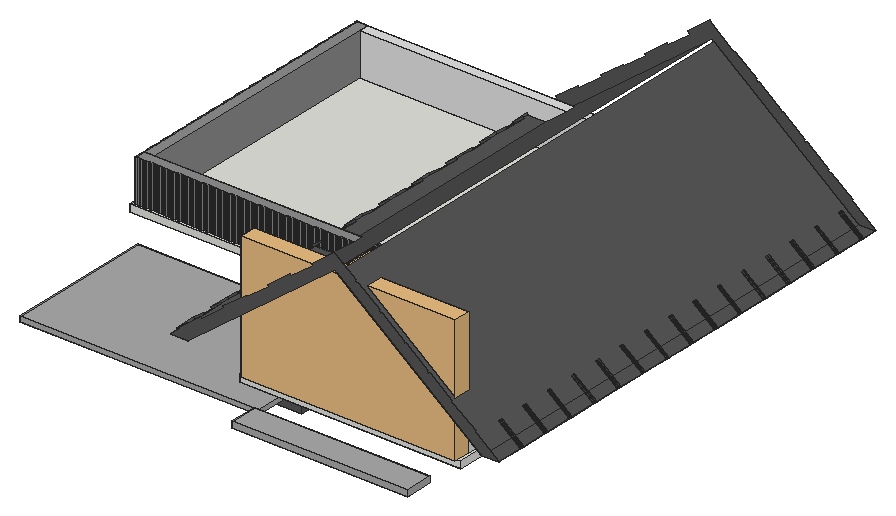
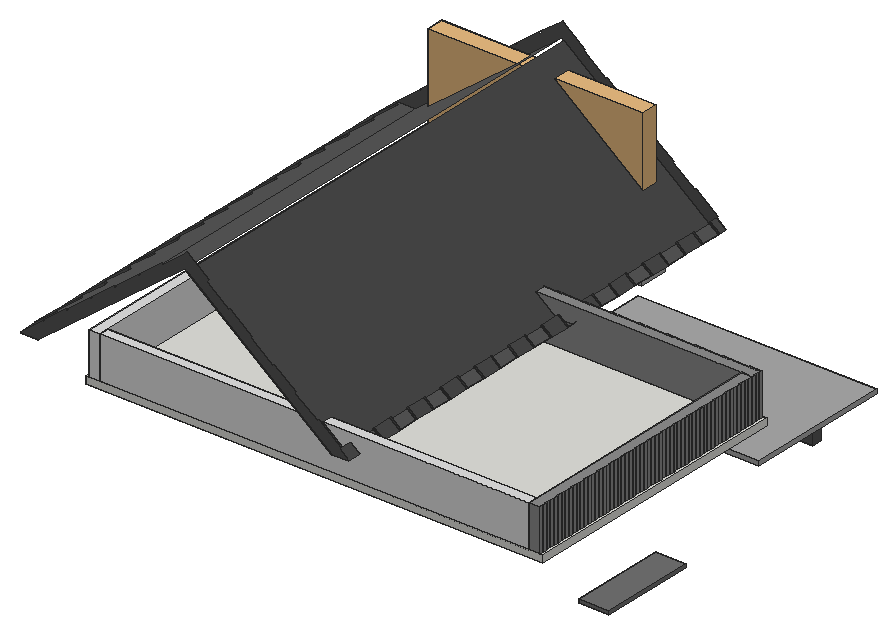
# SketchUp Ruby script. Lengths in inches.
U = 1.inch
M = Sketchup.active_model
def pt(a) = Geom::Point3d.new(a.map { |v| v * U })
def face(e, loops, mat)
  f = e.add_face(loops[0].map { |a| pt(a) })
  loops[1..].each { |l| e.add_face(l.map { |a| pt(a) }).erase! }
  f.material = f.back_material = mat if mat
  f
end
# faces: each face lists its corners as indices into pts; further lists are holes
def faces(e, pts, list, mat = nil) = list.each { |f| face(e, (f[0].is_a?(Array) ? f : [f]).map { |l| l.map { |i| pts[i] } }, mat) }
# xy, xz, yz: faces in a plane at the given z, y or x. An outline is a flat list of corners, or four numbers for a rectangle; further outlines are holes
def ring(l) = l.size == 4 ? [[l[0], l[1]], [l[2], l[1]], [l[2], l[3]], [l[0], l[3]]] : l.each_slice(2).to_a
def flat(e, list, mat, &to3) = list.each { |f| face(e, (f[0].is_a?(Array) ? f : [f]).map { |l| ring(l).map { |u, v| to3.(u, v) } }, mat) }
def xy(e, z, list, mat = nil) = flat(e, list, mat) { |x, y| [x, y, z] }
def xz(e, y, list, mat = nil) = flat(e, list, mat) { |x, z| [x, y, z] }
def yz(e, x, list, mat = nil) = flat(e, list, mat) { |y, z| [x, y, z] }
def lines(e, pts, list) = list.each { |a, b| e.add_line(pt(pts[a]), pt(pts[b])) }
# prism: a flat outline (further loops are holes) pulled along v
def prism(e, loops, v, mat = nil)
  f = face(e, loops, mat); d = Geom::Vector3d.new(v.map { |x| x * U })
  f.pushpull(f.normal.samedirection?(d) ? d.length : -d.length)
end
def box(e, o, s, mat = nil) = prism(e, [[o, [o[0] + s[0], o[1], o[2]], [o[0] + s[0], o[1] + s[1], o[2]], [o[0], o[1] + s[1], o[2]]]], [0, 0, s[2]], mat)
def at(x, y, z, deg = 0) = Geom::Transformation.translation(pt([x, y, z])) * Geom::Transformation.rotation(ORIGIN, Z_AXIS, deg.degrees)
def axes(o, x, y, z) = Geom::Transformation.new([*x, 0, *y, 0, *z, 0, *pt(o).to_a, 1])
def part(name) = M.definitions.add(name)
# library, detail: a bought-in or finely detailed component or shape, given as its bounding box
def library(name, o, s) = part(name).tap { |d| box(d.entities, o, s) }
def detail(e, o, s) = box(e.add_group.entities, o, s)
def put(e, d, t, mat = nil) = e.add_instance(d, t).tap { |i| i.material = mat if mat }
def group(e, t, mat = nil) = e.add_group.tap { |g| g.transformation = t; g.material = mat if mat }.entities
root = M.entities
M.materials.add("[Color M01]").color = [226, 226, 226]
M.materials.add("[Color M03]").color = [170, 170, 170]
M.materials.add("[Color M04]").color = [142, 142, 142]
M.materials.add("[Color M05]").color = [114, 114, 114]
M.materials.add("[Color M06]").color = [86, 86, 86]
c1 = library("Group\#80",[0,-5.8,-36],[184,14.8,108])
c2 = library("Group\#83",[-0.5,0,0],[9.5,135,36])
xy(root,328.19,[[236.86,137.375,251.46,541.1875],[503.2,137.375,517.81,541.1875]],"[Color M06]")
xz(root,137.375,[[236.86,328.19,251.46,328.19,375.48,425.25,377.33,426.7,379.18,425.25,503.2,328.19,517.81,328.19,518.42,328.98,499.52,343.77,498.91,342.98,497.33,344.21,497.95,345,479.05,359.79,478.43,359.01,476.86,360.24,477.47,361.03,458.57,375.82,457.95,375.03,456.38,376.26,457,377.05,438.1,391.84,437.48,391.05,435.9,392.29,436.52,393.07,417.62,407.87,417,407.08,415.43,408.3125,416.05,409.1,397.15,423.89,396.53,423.1,394.95,424.33,395.57,425.12,377.95,438.91,377.09,439.59,376.53,439.15,357.63,424.36,358.43,423.34,339.53,408.54,338.73,409.57,319.83,394.78,320.63,393.75,301.73,378.96,300.93,379.98,282.03,365.19,282.83,364.17,263.93,349.38,263.13,350.4,244.23,335.61,245.03,334.59]],"[Color M06]")
xz(root,145.1875,[[236.86,328.19,245.03,334.59,244.23,335.61,236.06,329.21]],"[Color M06]")
xz(root,161.375,[[517.81,328.19,498.91,342.98,499.52,343.77,518.42,328.98]],"[Color M06]")
xz(root,163.1875,[[236.86,328.19,236.06,329.21,244.23,335.61,245.03,334.59]],"[Color M06]")
xz(root,163.375,[[517.81,328.19,518.42,328.98,499.52,343.77,498.91,342.98]],"[Color M06]")
xz(root,181.1875,[[236.86,328.19,245.03,334.59,244.54,335.22,244.23,335.61,236.06,329.21]],"[Color M06]")
xz(root,187.375,[[517.81,328.19,498.91,342.98,499.52,343.77,518.42,328.98]],"[Color M06]")
xz(root,189.375,[[517.81,328.19,518.42,328.98,499.52,343.77,498.91,342.98]],"[Color M06]")
xz(root,199.1875,[[236.86,328.19,236.06,329.21,244.23,335.61,244.54,335.22,245.03,334.59]],"[Color M06]")
xz(root,213.375,[[517.81,328.19,498.91,342.98,499.52,343.77,518.42,328.98]],"[Color M06]")
xz(root,215.375,[[517.81,328.19,518.42,328.98,499.52,343.77,498.91,342.98]],"[Color M06]")
xz(root,217.1875,[[236.86,328.19,245.03,334.59,244.54,335.22,244.23,335.61,236.06,329.21]],"[Color M06]")
xz(root,235.1875,[[236.86,328.19,236.06,329.21,244.23,335.61,244.54,335.22,245.03,334.59]],"[Color M06]")
xz(root,239.375,[[517.81,328.19,498.91,342.98,499.52,343.77,518.42,328.98]],"[Color M06]")
xz(root,241.375,[[517.81,328.19,518.42,328.98,499.52,343.77,498.91,342.98]],"[Color M06]")
xz(root,253.1875,[[236.86,328.19,245.03,334.59,244.23,335.61,236.06,329.21]],"[Color M06]")
xz(root,265.375,[[517.81,328.19,498.91,342.98,499.52,343.77,518.42,328.98]],"[Color M06]")
xz(root,267.375,[[517.81,328.19,518.42,328.98,499.52,343.77,498.91,342.98]],"[Color M06]")
xz(root,271.1875,[[236.86,328.19,236.06,329.21,244.23,335.61,245.03,334.59]],"[Color M06]")
xz(root,289.1875,[[236.86,328.19,245.03,334.59,244.54,335.22,244.23,335.61,236.06,329.21]],"[Color M06]")
xz(root,291.375,[[517.81,328.19,498.91,342.98,499.52,343.77,518.42,328.98]],"[Color M06]")
xz(root,293.375,[[517.81,328.19,518.42,328.98,499.52,343.77,498.91,342.98]],"[Color M06]")
xz(root,307.1875,[[236.86,328.19,236.06,329.21,244.23,335.61,244.54,335.22,245.03,334.59]],"[Color M06]")
xz(root,317.375,[[517.81,328.19,498.91,342.98,499.52,343.77,518.42,328.98]],"[Color M06]")
xz(root,319.375,[[517.81,328.19,518.42,328.98,499.52,343.77,498.91,342.98]],"[Color M06]")
xz(root,325.1875,[[236.86,328.19,245.03,334.59,244.54,335.22,244.23,335.61,236.06,329.21]],"[Color M06]")
xz(root,343.1875,[[236.86,328.19,236.06,329.21,244.23,335.61,244.54,335.22,245.03,334.59]],"[Color M06]")
xz(root,343.375,[[517.81,328.19,498.91,342.98,499.52,343.77,518.42,328.98]],"[Color M06]")
xz(root,345.375,[[517.81,328.19,518.42,328.98,499.52,343.77,498.91,342.98]],"[Color M06]")
xz(root,361.1875,[[236.86,328.19,245.03,334.59,244.54,335.22,244.23,335.61,236.06,329.21]],"[Color M06]")
xz(root,369.375,[[517.81,328.19,498.91,342.98,499.52,343.77,518.42,328.98]],"[Color M06]")
xz(root,371.375,[[517.81,328.19,518.42,328.98,499.52,343.77,498.91,342.98]],"[Color M06]")
xz(root,379.1875,[[236.86,328.19,236.06,329.21,244.23,335.61,244.54,335.22,245.03,334.59]],"[Color M06]")
xz(root,395.375,[[517.81,328.19,498.91,342.98,499.52,343.77,518.42,328.98]],"[Color M06]")
xz(root,397.1875,[[236.86,328.19,245.03,334.59,244.23,335.61,236.06,329.21]],"[Color M06]")
xz(root,397.375,[[517.81,328.19,518.42,328.98,499.52,343.77,498.91,342.98]],"[Color M06]")
xz(root,415.1875,[[236.86,328.19,236.06,329.21,244.23,335.61,245.03,334.59]],"[Color M06]")
xz(root,421.375,[[517.81,328.19,498.91,342.98,499.52,343.77,518.42,328.98]],"[Color M06]")
xz(root,423.375,[[517.81,328.19,518.42,328.98,499.52,343.77,498.91,342.98]],"[Color M06]")
xz(root,433.1875,[[236.86,328.19,245.03,334.59,244.23,335.61,236.06,329.21]],"[Color M06]")
xz(root,447.375,[[517.81,328.19,498.91,342.98,499.52,343.77,518.42,328.98]],"[Color M06]")
xz(root,449.375,[[517.81,328.19,518.42,328.98,499.52,343.77,498.91,342.98]],"[Color M06]")
xz(root,451.1875,[[236.86,328.19,236.06,329.21,244.23,335.61,245.03,334.59]],"[Color M06]")
xz(root,469.1875,[[236.86,328.19,245.03,334.59,244.54,335.22,244.23,335.61,236.06,329.21]],"[Color M06]")
xz(root,473.375,[[517.81,328.19,498.91,342.98,499.52,343.77,518.42,328.98]],"[Color M06]")
xz(root,475.375,[[517.81,328.19,518.42,328.98,499.52,343.77,498.91,342.98]],"[Color M06]")
xz(root,487.1875,[[236.86,328.19,236.06,329.21,244.23,335.61,244.54,335.22,245.03,334.59]],"[Color M06]")
xz(root,499.375,[[517.81,328.19,498.91,342.98,499.52,343.77,518.42,328.98]],"[Color M06]")
xz(root,501.375,[[517.81,328.19,518.42,328.98,499.52,343.77,498.91,342.98]],"[Color M06]")
xz(root,505.1875,[[236.86,328.19,245.03,334.59,244.54,335.22,244.23,335.61,236.06,329.21]],"[Color M06]")
xz(root,523.1875,[[236.86,328.19,236.06,329.21,244.23,335.61,244.54,335.22,245.03,334.59]],"[Color M06]")
xz(root,525.375,[[517.81,328.19,498.91,342.98,499.52,343.77,518.42,328.98]],"[Color M06]")
xz(root,527.375,[[517.81,328.19,518.42,328.98,499.52,343.77,498.91,342.98]],"[Color M06]")
xz(root,541.1875,[[236.86,328.19,245.03,334.59,244.18,335.67,263.08,350.46,263.93,349.38,282.83,364.17,281.98,365.25,300.88,380.04,301.73,378.96,320.63,393.75,319.78,394.84,338.68,409.625,339.53,408.54,358.43,423.34,356.78,425.44,375.68,440.23,376.53,439.15,377.33,438.125,394.95,424.33,396.53,423.1,397.15,423.89,416.05,409.1,415.43,408.3125,417,407.08,417.62,407.87,436.52,393.07,435.9,392.29,437.48,391.05,438.1,391.84,457,377.05,456.38,376.26,457.95,375.03,458.57,375.82,477.47,361.03,476.86,360.24,478.43,359.01,479.05,359.79,497.95,345,497.33,344.21,498.91,342.98,499.52,343.77,518.42,328.98,517.81,328.19,503.2,328.19,379.18,425.25,377.33,426.7,375.48,425.25,251.46,328.19]],"[Color M06]")
p = [[236.86,137.375,328.19],[245.03,137.375,334.59],[245.03,145.1875,334.59],[236.86,145.1875,328.19],[375.48,137.375,425.25],[251.46,137.375,328.19],
  [251.46,541.1875,328.19],[375.48,541.1875,425.25],[503.2,541.1875,328.19],[503.2,137.375,328.19],[379.18,137.375,425.25],[379.18,541.1875,425.25],
  [517.81,137.375,328.19],[517.81,161.375,328.19],[518.42,161.375,328.98],[518.42,137.375,328.98],[236.86,163.1875,328.19],[236.06,145.1875,329.21],
  [236.06,163.1875,329.21],[517.81,163.375,328.19],[498.91,163.375,342.98],[498.91,161.375,342.98],[245.03,163.1875,334.59],[245.03,181.1875,334.59],
  [236.86,181.1875,328.19],[517.81,187.375,328.19],[518.42,187.375,328.98],[518.42,163.375,328.98],[236.86,199.1875,328.19],[236.06,181.1875,329.21],
  [236.06,199.1875,329.21],[517.81,189.375,328.19],[498.91,189.375,342.98],[498.91,187.375,342.98],[517.81,213.375,328.19],[518.42,213.375,328.98],
  [518.42,189.375,328.98],[245.03,199.1875,334.59],[245.03,217.1875,334.59],[236.86,217.1875,328.19],[517.81,215.375,328.19],[498.91,215.375,342.98],
  [498.91,213.375,342.98],[517.81,239.375,328.19],[518.42,239.375,328.98],[518.42,215.375,328.98],[236.86,235.1875,328.19],[236.06,217.1875,329.21],
  [236.06,235.1875,329.21],[245.03,235.1875,334.59],[245.03,253.1875,334.59],[236.86,253.1875,328.19],[517.81,241.375,328.19],[498.91,241.375,342.98],
  [498.91,239.375,342.98],[517.81,265.375,328.19],[518.42,265.375,328.98],[518.42,241.375,328.98],[236.86,271.1875,328.19],[236.06,253.1875,329.21],
  [236.06,271.1875,329.21],[517.81,267.375,328.19],[498.91,267.375,342.98],[498.91,265.375,342.98],[517.81,291.375,328.19],[518.42,291.375,328.98],
  [518.42,267.375,328.98],[245.03,271.1875,334.59],[245.03,289.1875,334.59],[236.86,289.1875,328.19],[236.86,307.1875,328.19],[236.06,289.1875,329.21],
  [236.06,307.1875,329.21],[517.81,293.375,328.19],[498.91,293.375,342.98],[498.91,291.375,342.98],[517.81,317.375,328.19],[518.42,317.375,328.98],
  [518.42,293.375,328.98],[245.03,307.1875,334.59],[245.03,325.1875,334.59],[236.86,325.1875,328.19],[517.81,319.375,328.19],[498.91,319.375,342.98],
  [498.91,317.375,342.98],[517.81,343.375,328.19],[518.42,343.375,328.98],[518.42,319.375,328.98],[236.86,343.1875,328.19],[236.06,325.1875,329.21],
  [236.06,343.1875,329.21],[245.03,343.1875,334.59],[245.03,361.1875,334.59],[236.86,361.1875,328.19],[517.81,345.375,328.19],[498.91,345.375,342.98],
  [498.91,343.375,342.98],[517.81,369.375,328.19],[518.42,369.375,328.98],[518.42,345.375,328.98],[236.86,379.1875,328.19],[236.06,361.1875,329.21],
  [236.06,379.1875,329.21],[517.81,371.375,328.19],[498.91,371.375,342.98],[498.91,369.375,342.98],[517.81,395.375,328.19],[518.42,395.375,328.98],
  [518.42,371.375,328.98],[245.03,379.1875,334.59],[245.03,397.1875,334.59],[236.86,397.1875,328.19],[517.81,397.375,328.19],[498.91,397.375,342.98],
  [498.91,395.375,342.98],[236.86,415.1875,328.19],[236.06,397.1875,329.21],[236.06,415.1875,329.21],[517.81,421.375,328.19],[518.42,421.375,328.98],
  [518.42,397.375,328.98],[245.03,415.1875,334.59],[245.03,433.1875,334.59],[236.86,433.1875,328.19],[517.81,423.375,328.19],[498.91,423.375,342.98],
  [498.91,421.375,342.98],[517.81,447.375,328.19],[518.42,447.375,328.98],[518.42,423.375,328.98],[236.86,451.1875,328.19],[236.06,433.1875,329.21],
  [236.06,451.1875,329.21],[517.81,449.375,328.19],[498.91,449.375,342.98],[498.91,447.375,342.98],[517.81,473.375,328.19],[518.42,473.375,328.98],
  [518.42,449.375,328.98],[245.03,451.1875,334.59],[245.03,469.1875,334.59],[236.86,469.1875,328.19],[236.86,487.1875,328.19],[236.06,469.1875,329.21],
  [236.06,487.1875,329.21],[517.81,475.375,328.19],[498.91,475.375,342.98],[498.91,473.375,342.98],[517.81,499.375,328.19],[518.42,499.375,328.98],
  [518.42,475.375,328.98],[245.03,487.1875,334.59],[245.03,505.1875,334.59],[236.86,505.1875,328.19],[517.81,501.375,328.19],[498.91,501.375,342.98],
  [498.91,499.375,342.98],[517.81,525.375,328.19],[518.42,525.375,328.98],[518.42,501.375,328.98],[236.86,523.1875,328.19],[236.06,505.1875,329.21],
  [236.06,523.1875,329.21],[245.03,523.1875,334.59],[245.03,541.1875,334.59],[236.86,541.1875,328.19],[517.81,527.375,328.19],[498.91,527.375,342.98],
  [498.91,525.375,342.98],[517.81,541.1875,328.19],[518.42,541.1875,328.98],[518.42,527.375,328.98]]
faces(root,p,[[0,1,2,3],[4,5,6,7],[8,9,10,11],[12,13,14,15],[16,3,17,18],[19,20,21,13],[16,22,23,24],[19,25,26,27],
  [28,24,29,30],[31,32,33,25],[31,34,35,36],[28,37,38,39],[40,41,42,34],[40,43,44,45],[46,39,47,48],[46,49,50,51],
  [52,53,54,43],[52,55,56,57],[58,51,59,60],[61,62,63,55],[61,64,65,66],[58,67,68,69],[70,69,71,72],[73,74,75,64],
  [73,76,77,78],[70,79,80,81],[82,83,84,76],[82,85,86,87],[88,81,89,90],[88,91,92,93],[94,95,96,85],[94,97,98,99],
  [100,93,101,102],[103,104,105,97],[103,106,107,108],[100,109,110,111],[112,113,114,106],[115,111,116,117],[112,118,119,120],[115,121,122,123],
  [124,125,126,118],[124,127,128,129],[130,123,131,132],[133,134,135,127],[133,136,137,138],[130,139,140,141],[142,141,143,144],[145,146,147,136],
  [145,148,149,150],[142,151,152,153],[154,155,156,148],[154,157,158,159],[160,153,161,162],[160,163,164,165],[166,167,168,157],[166,169,170,171]],"[Color M06]")
g1 = group(root,at(59.33,402.375,248),"[Color M05]")
box(g1,[0,0,0],[26,82,3])
g2 = group(root,at(94.33,214.375,250.375),"[Color M06]")
box(g2,[0,0,0],[193,7.75,9.625])
g3 = group(root,at(85.33,177.375,270),"[Color M03]")
box(g3,[-2,-9,0],[204,126,4])
g4 = group(root,at(291.33,135.375,276),"[Color M03]")
box(g4,[0,0,0],[150,24,5])
g5 = group(root,at(80.33,154.375,300))
prism(g5,[[[0,135,0],[0,374.8125,0],[392,374.8125,0],[392,0,0],[202,0,0],[202,135,0]]],[0,0,6])
g6 = group(root,at(83.33,301.375,306),"[Color M04]")
prism(g6,[[[9,227.8125,0],[9,0,0],[0,0,0],[0,1.8125,0],[-0.5,1.8125,0],[-0.5,3.8125,0],[0,3.8125,0],[0,5.8125,0],[-0.5,5.8125,0],[-0.5,7.8125,0],[0,7.8125,0],[0,9.8125,0],[-0.5,9.8125,0],[-0.5,11.8125,0],[0,11.8125,0],[0,13.8125,0],[-0.5,13.8125,0],[-0.5,15.8125,0],[0,15.8125,0],[0,17.8125,0],[-0.5,17.8125,0],[-0.5,19.8125,0],[0,19.8125,0],[0,21.8125,0],[-0.5,21.8125,0],[-0.5,23.8125,0],[0,23.8125,0],[0,25.8125,0],[-0.5,25.8125,0],[-0.5,27.8125,0],[0,27.8125,0],[0,29.8125,0],[-0.5,29.8125,0],[-0.5,31.8125,0],[0,31.8125,0],[0,33.8125,0],[-0.5,33.8125,0],[-0.5,35.8125,0],[0,35.8125,0],[0,37.8125,0],[-0.5,37.8125,0],[-0.5,39.8125,0],[0,39.8125,0],[0,41.8125,0],[-0.5,41.8125,0],[-0.5,43.8125,0],[0,43.8125,0],[0,45.8125,0],[-0.5,45.8125,0],[-0.5,47.8125,0],[0,47.8125,0],[0,49.8125,0],[-0.5,49.8125,0],[-0.5,51.8125,0],[0,51.8125,0],[0,53.8125,0],[-0.5,53.8125,0],[-0.5,55.8125,0],[0,55.8125,0],[0,57.8125,0],[-0.5,57.8125,0],[-0.5,59.8125,0],[0,59.8125,0],[0,61.8125,0],[-0.5,61.8125,0],[-0.5,63.8125,0],[0,63.8125,0],[0,65.8125,0],[-0.5,65.8125,0],[-0.5,67.8125,0],[0,67.8125,0],[0,69.8125,0],[-0.5,69.8125,0],[-0.5,71.8125,0],[0,71.8125,0],[0,73.8125,0],[-0.5,73.8125,0],[-0.5,75.8125,0],[0,75.8125,0],[0,77.8125,0],[-0.5,77.8125,0],[-0.5,79.8125,0],[0,79.8125,0],[0,81.8125,0],[-0.5,81.8125,0],[-0.5,83.8125,0],[0,83.8125,0],[0,85.8125,0],[-0.5,85.8125,0],[-0.5,87.8125,0],[0,87.8125,0],[0,89.8125,0],[-0.5,89.8125,0],[-0.5,91.8125,0],[0,91.8125,0],[0,93.8125,0],[-0.5,93.8125,0],[-0.5,95.8125,0],[0,95.8125,0],[0,97.8125,0],[-0.5,97.8125,0],[-0.5,99.8125,0],[0,99.8125,0],[0,101.8125,0],[-0.5,101.8125,0],[-0.5,103.8125,0],[0,103.8125,0],[0,105.8125,0],[-0.5,105.8125,0],[-0.5,107.8125,0],[0,107.8125,0],[0,109.8125,0],[-0.5,109.8125,0],[-0.5,111.8125,0],[0,111.8125,0],[0,113.8125,0],[-0.5,113.8125,0],[-0.5,115.8125,0],[0,115.8125,0],[0,117.8125,0],[-0.5,117.8125,0],[-0.5,119.8125,0],[0,119.8125,0],[0,121.8125,0],[-0.5,121.8125,0],[-0.5,123.8125,0],[0,123.8125,0],[0,125.8125,0],[-0.5,125.8125,0],[-0.5,127.8125,0],[0,127.8125,0],[0,129.8125,0],[-0.5,129.8125,0],[-0.5,131.8125,0],[0,131.8125,0],[0,133.8125,0],[-0.5,133.8125,0],[-0.5,135.8125,0],[0,135.8125,0],[0,137.8125,0],[-0.5,137.8125,0],[-0.5,139.8125,0],[0,139.8125,0],[0,141.8125,0],[-0.5,141.8125,0],[-0.5,143.8125,0],[0,143.8125,0],[0,145.8125,0],[-0.5,145.8125,0],[-0.5,147.8125,0],[0,147.8125,0],[0,149.8125,0],[-0.5,149.8125,0],[-0.5,151.8125,0],[0,151.8125,0],[0,153.8125,0],[-0.5,153.8125,0],[-0.5,155.8125,0],[0,155.8125,0],[0,157.8125,0],[-0.5,157.8125,0],[-0.5,159.8125,0],[0,159.8125,0],[0,161.8125,0],[-0.5,161.8125,0],[-0.5,163.8125,0],[0,163.8125,0],[0,165.8125,0],[-0.5,165.8125,0],[-0.5,167.8125,0],[0,167.8125,0],[0,169.8125,0],[-0.5,169.8125,0],[-0.5,171.8125,0],[0,171.8125,0],[0,173.8125,0],[-0.5,173.8125,0],[-0.5,175.8125,0],[0,175.8125,0],[0,177.8125,0],[-0.5,177.8125,0],[-0.5,179.8125,0],[0,179.8125,0],[0,181.8125,0],[-0.5,181.8125,0],[-0.5,183.8125,0],[0,183.8125,0],[0,185.8125,0],[-0.5,185.8125,0],[-0.5,187.8125,0],[0,187.8125,0],[0,189.8125,0],[-0.5,189.8125,0],[-0.5,191.8125,0],[0,191.8125,0],[0,193.8125,0],[-0.5,193.8125,0],[-0.5,195.8125,0],[0,195.8125,0],[0,197.8125,0],[-0.5,197.8125,0],[-0.5,199.8125,0],[0,199.8125,0],[0,201.8125,0],[-0.5,201.8125,0],[-0.5,203.8125,0],[0,203.8125,0],[0,205.8125,0],[-0.5,205.8125,0],[-0.5,207.8125,0],[0,207.8125,0],[0,209.8125,0],[-0.5,209.8125,0],[-0.5,211.8125,0],[0,211.8125,0],[0,213.8125,0],[-0.5,213.8125,0],[-0.5,215.8125,0],[0,215.8125,0],[0,217.8125,0],[-0.5,217.8125,0],[-0.5,219.8125,0],[0,219.8125,0],[0,221.8125,0],[-0.5,221.8125,0],[-0.5,223.8125,0],[0,223.8125,0],[0,225.8125,0],[-0.5,225.8125,0],[-0.5,227.8125,0]]],[0,0,36])
g7 = group(root,at(83.33,292.375,306),"[Color M04]")
prism(g7,[[[2,-0.5,0],[-0.5,-0.5,0],[-0.5,1,0],[0,1,0],[0,3,0],[-0.5,3,0],[-0.5,5,0],[0,5,0],[0,7,0],[-0.5,7,0],[-0.5,9,0],[202,9,0],[202,-0.5,0],[200,-0.5,0],[200,0,0],[198,0,0],[198,-0.5,0],[196,-0.5,0],[196,0,0],[194,0,0],[194,-0.5,0],[192,-0.5,0],[192,0,0],[190,0,0],[190,-0.5,0],[188,-0.5,0],[188,0,0],[186,0,0],[186,-0.5,0],[184,-0.5,0],[184,0,0],[182,0,0],[182,-0.5,0],[180,-0.5,0],[180,0,0],[178,0,0],[178,-0.5,0],[176,-0.5,0],[176,0,0],[174,0,0],[174,-0.5,0],[172,-0.5,0],[172,0,0],[170,0,0],[170,-0.5,0],[168,-0.5,0],[168,0,0],[166,0,0],[166,-0.5,0],[164,-0.5,0],[164,0,0],[162,0,0],[162,-0.5,0],[160,-0.5,0],[160,0,0],[158,0,0],[158,-0.5,0],[156,-0.5,0],[156,0,0],[154,0,0],[154,-0.5,0],[152,-0.5,0],[152,0,0],[150,0,0],[150,-0.5,0],[148,-0.5,0],[148,0,0],[146,0,0],[146,-0.5,0],[144,-0.5,0],[144,0,0],[142,0,0],[142,-0.5,0],[140,-0.5,0],[140,0,0],[138,0,0],[138,-0.5,0],[136,-0.5,0],[136,0,0],[134,0,0],[134,-0.5,0],[132,-0.5,0],[132,0,0],[130,0,0],[130,-0.5,0],[128,-0.5,0],[128,0,0],[126,0,0],[126,-0.5,0],[124,-0.5,0],[124,0,0],[122,0,0],[122,-0.5,0],[120,-0.5,0],[120,0,0],[118,0,0],[118,-0.5,0],[116,-0.5,0],[116,0,0],[114,0,0],[114,-0.5,0],[112,-0.5,0],[112,0,0],[110,0,0],[110,-0.5,0],[108,-0.5,0],[108,0,0],[106,0,0],[106,-0.5,0],[104,-0.5,0],[104,0,0],[102,0,0],[102,-0.5,0],[100,-0.5,0],[100,0,0],[98,0,0],[98,-0.5,0],[96,-0.5,0],[96,0,0],[94,0,0],[94,-0.5,0],[92,-0.5,0],[92,0,0],[90,0,0],[90,-0.5,0],[88,-0.5,0],[88,0,0],[86,0,0],[86,-0.5,0],[84,-0.5,0],[84,0,0],[82,0,0],[82,-0.5,0],[80,-0.5,0],[80,0,0],[78,0,0],[78,-0.5,0],[76,-0.5,0],[76,0,0],[74,0,0],[74,-0.5,0],[72,-0.5,0],[72,0,0],[70,0,0],[70,-0.5,0],[68,-0.5,0],[68,0,0],[66,0,0],[66,-0.5,0],[64,-0.5,0],[64,0,0],[62,0,0],[62,-0.5,0],[60,-0.5,0],[60,0,0],[58,0,0],[58,-0.5,0],[56,-0.5,0],[56,0,0],[54,0,0],[54,-0.5,0],[52,-0.5,0],[52,0,0],[50,0,0],[50,-0.5,0],[48,-0.5,0],[48,0,0],[46,0,0],[46,-0.5,0],[44,-0.5,0],[44,0,0],[42,0,0],[42,-0.5,0],[40,-0.5,0],[40,0,0],[38,0,0],[38,-0.5,0],[36,-0.5,0],[36,0,0],[34,0,0],[34,-0.5,0],[32,-0.5,0],[32,0,0],[30,0,0],[30,-0.5,0],[28,-0.5,0],[28,0,0],[26,0,0],[26,-0.5,0],[24,-0.5,0],[24,0,0],[22,0,0],[22,-0.5,0],[20,-0.5,0],[20,0,0],[18,0,0],[18,-0.5,0],[16,-0.5,0],[16,0,0],[14,0,0],[14,-0.5,0],[12,-0.5,0],[12,0,0],[10,0,0],[10,-0.5,0],[8,-0.5,0],[8,0,0],[6,0,0],[6,-0.5,0],[4,-0.5,0],[4,0,0],[2,0,0]]],[0,0,36])
put(root,c1,at(285.33,157.375,342),"[Color M04]")
g8 = group(root,at(460.33,166.375,306),"[Color M01]")
box(g8,[0,0,0],[9,362.8125,36])
g9 = group(root,at(92.33,520.1875,306),"[Color M01]")
box(g9,[0,0,0],[368,9,36])
put(root,c2,at(285.33,166.375,306),"[Color M04]")
